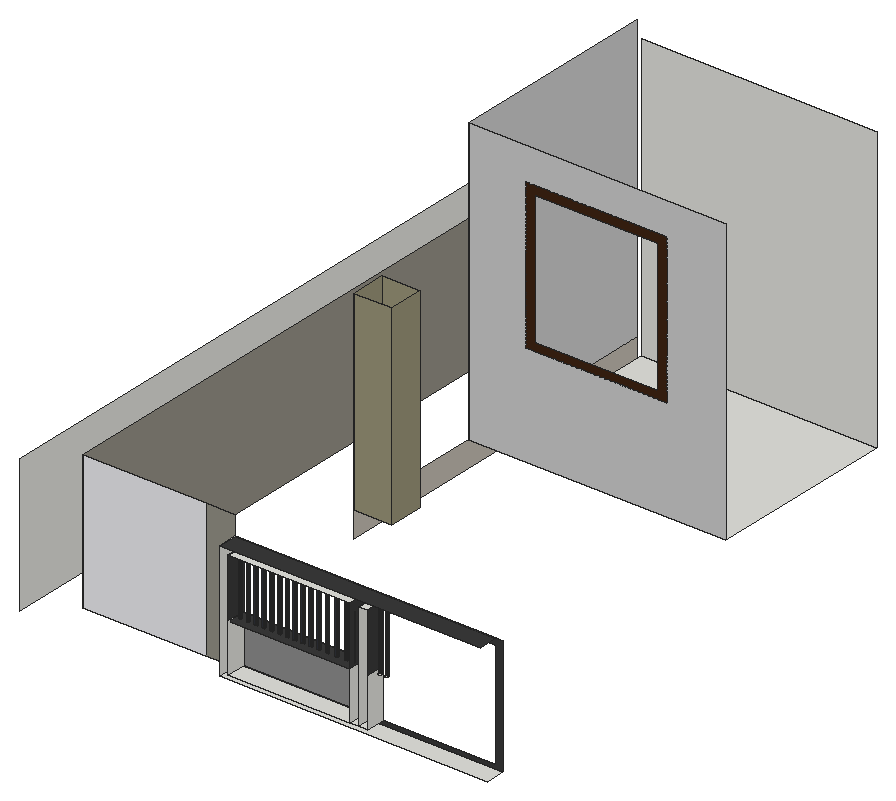
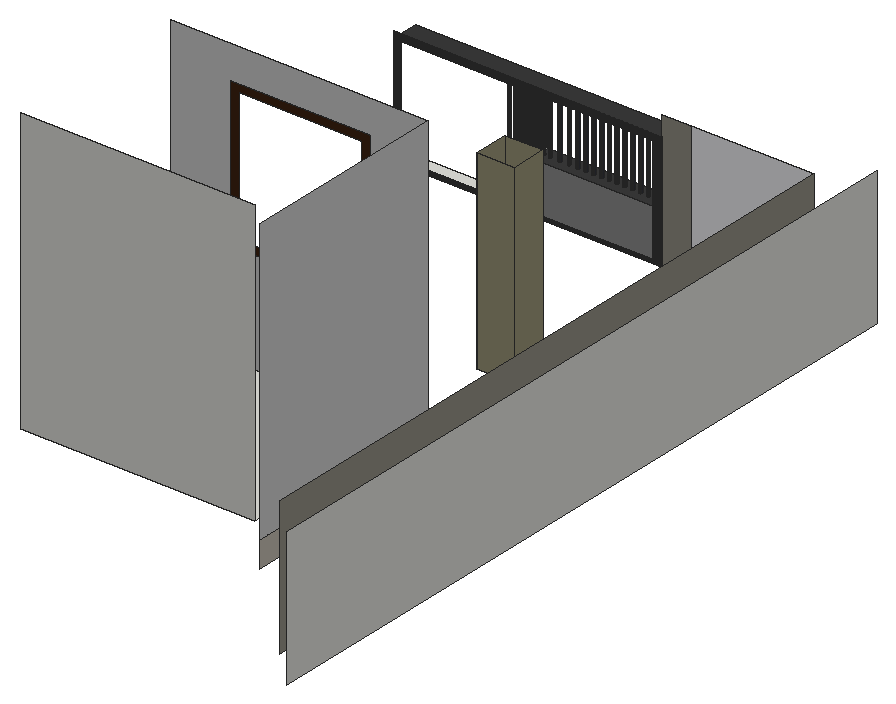
# SketchUp Ruby script. Lengths in inches.
U = 1.inch
M = Sketchup.active_model
def pt(a) = Geom::Point3d.new(a.map { |v| v * U })
def face(e, loops, mat)
  f = e.add_face(loops[0].map { |a| pt(a) })
  loops[1..].each { |l| e.add_face(l.map { |a| pt(a) }).erase! }
  f.material = f.back_material = mat if mat
  f
end
# faces: each face lists its corners as indices into pts; further lists are holes
def faces(e, pts, list, mat = nil) = list.each { |f| face(e, (f[0].is_a?(Array) ? f : [f]).map { |l| l.map { |i| pts[i] } }, mat) }
# xy, xz, yz: faces in a plane at the given z, y or x. An outline is a flat list of corners, or four numbers for a rectangle; further outlines are holes
def ring(l) = l.size == 4 ? [[l[0], l[1]], [l[2], l[1]], [l[2], l[3]], [l[0], l[3]]] : l.each_slice(2).to_a
def flat(e, list, mat, &to3) = list.each { |f| face(e, (f[0].is_a?(Array) ? f : [f]).map { |l| ring(l).map { |u, v| to3.(u, v) } }, mat) }
def xy(e, z, list, mat = nil) = flat(e, list, mat) { |x, y| [x, y, z] }
def xz(e, y, list, mat = nil) = flat(e, list, mat) { |x, z| [x, y, z] }
def yz(e, x, list, mat = nil) = flat(e, list, mat) { |y, z| [x, y, z] }
def lines(e, pts, list) = list.each { |a, b| e.add_line(pt(pts[a]), pt(pts[b])) }
# prism: a flat outline (further loops are holes) pulled along v
def prism(e, loops, v, mat = nil)
  f = face(e, loops, mat); d = Geom::Vector3d.new(v.map { |x| x * U })
  f.pushpull(f.normal.samedirection?(d) ? d.length : -d.length)
end
def box(e, o, s, mat = nil) = prism(e, [[o, [o[0] + s[0], o[1], o[2]], [o[0] + s[0], o[1] + s[1], o[2]], [o[0], o[1] + s[1], o[2]]]], [0, 0, s[2]], mat)
def at(x, y, z, deg = 0) = Geom::Transformation.translation(pt([x, y, z])) * Geom::Transformation.rotation(ORIGIN, Z_AXIS, deg.degrees)
def axes(o, x, y, z) = Geom::Transformation.new([*x, 0, *y, 0, *z, 0, *pt(o).to_a, 1])
def part(name) = M.definitions.add(name)
# library, detail: a bought-in or finely detailed component or shape, given as its bounding box
def library(name, o, s) = part(name).tap { |d| box(d.entities, o, s) }
def detail(e, o, s) = box(e.add_group.entities, o, s)
def put(e, d, t, mat = nil) = e.add_instance(d, t).tap { |i| i.material = mat if mat }
def group(e, t, mat = nil) = e.add_group.tap { |g| g.transformation = t; g.material = mat if mat }.entities
root = M.entities
M.materials.add("[Blinds Vertical Pattern]1").color = [239, 239, 242]
M.materials.add("[Cladding Siding White]").color = [207, 207, 207]
M.materials.add("[Color M04]").color = [142, 142, 142]
M.materials.add("[Color M07]").color = [58, 58, 58]
M.materials.add("[Field Rectangle Tile]").color = [196, 189, 179]
M.materials.add("[Formica Graystone]").color = [149, 146, 135]
M.materials.add("[Formica Laminate Dark]").color = [50, 53, 60]
M.materials.add("[Stone Coursed Rough]").color = [155, 150, 122]
M.materials.add("[Wood Veneer 01]").color = [63, 37, 19]
xy(root,0,[[79.1,102.91,192.64,111]])
xy(root,1.75,[[82.65,102.91,134.27,111],[134.27,102.91,138.0625,111],[138.0625,102.91,141.86,111]])
xy(root,10.875,[[55.77,203.17,71.76,217.98],[64.9,263.99,164.37,343.79]])
xy(root,22.1875,[[132.58,106,132.4,106.02,132.24,106.09,132.1,106.2,131.99,106.34,131.92,106.51,131.9,106.6875,131.92,106.87,131.99,107.03,132.1,107.17,132.24,107.28,132.4,107.35,132.58,107.375,132.76,107.35,132.93,107.28,133.07,107.17,133.18,107.03,133.25,106.87,133.27,106.6875,133.25,106.51,133.18,106.34,133.07,106.2,132.93,106.09,132.76,106.02],[144.08,106,143.9,106.02,143.74,106.09,143.6,106.2,143.49,106.34,143.42,106.51,143.4,106.6875,143.42,106.87,143.49,107.03,143.6,107.17,143.74,107.28,143.9,107.35,144.08,107.375,144.26,107.35,144.43,107.28,144.57,107.17,144.68,107.03,144.75,106.87,144.77,106.6875,144.75,106.51,144.68,106.34,144.57,106.2,144.43,106.09,144.26,106.02],[146.96,106,146.78,106.02,146.61,106.09,146.47,106.2,146.36,106.34,146.29,106.51,146.27,106.6875,146.29,106.87,146.36,107.03,146.47,107.17,146.61,107.28,146.78,107.35,146.96,107.375,147.14,107.35,147.3,107.28,147.44,107.17,147.55,107.03,147.62,106.87,147.65,106.6875,147.62,106.51,147.55,106.34,147.44,106.2,147.3,106.09,147.14,106.02]])
xy(root,22.1875,[[[82.65,102.91,134.27,111],[88.02,106,87.84,106.02,87.68,106.09,87.53,106.2,87.42,106.34,87.36,106.51,87.33,106.6875,87.36,106.87,87.42,107.03,87.53,107.17,87.68,107.28,87.84,107.35,88.02,107.375,88.2,107.35,88.36,107.28,88.51,107.17,88.62,107.03,88.68,106.87,88.71,106.6875,88.68,106.51,88.62,106.34,88.51,106.2,88.36,106.09,88.2,106.02],[91.33,106,91.15,106.02,90.99,106.09,90.85,106.2,90.74,106.34,90.67,106.51,90.65,106.6875,90.67,106.87,90.74,107.03,90.85,107.17,90.99,107.28,91.15,107.35,91.33,107.375,91.51,107.35,91.68,107.28,91.82,107.17,91.93,107.03,92,106.87,92.02,106.6875,92,106.51,91.93,106.34,91.82,106.2,91.68,106.09,91.51,106.02],[94.65,106,94.47,106.02,94.3,106.09,94.16,106.2,94.05,106.34,93.98,106.51,93.96,106.6875,93.98,106.87,94.05,107.03,94.16,107.17,94.3,107.28,94.47,107.35,94.65,107.375,94.82,107.35,94.99,107.28,95.13,107.17,95.24,107.03,95.31,106.87,95.33,106.6875,95.31,106.51,95.24,106.34,95.13,106.2,94.99,106.09,94.82,106.02],[97.96,106,97.78,106.02,97.61,106.09,97.47,106.2,97.36,106.34,97.29,106.51,97.27,106.6875,97.29,106.87,97.36,107.03,97.47,107.17,97.61,107.28,97.78,107.35,97.96,107.375,98.14,107.35,98.3,107.28,98.44,107.17,98.55,107.03,98.62,106.87,98.65,106.6875,98.62,106.51,98.55,106.34,98.44,106.2,98.3,106.09,98.14,106.02],[101.27,106,101.09,106.02,100.93,106.09,100.78,106.2,100.67,106.34,100.61,106.51,100.58,106.6875,100.61,106.87,100.67,107.03,100.78,107.17,100.93,107.28,101.09,107.35,101.27,107.375,101.45,107.35,101.61,107.28,101.76,107.17,101.87,107.03,101.93,106.87,101.96,106.6875,101.93,106.51,101.87,106.34,101.76,106.2,101.61,106.09,101.45,106.02],[104.58,106,104.4,106.02,104.24,106.09,104.1,106.2,103.99,106.34,103.92,106.51,103.9,106.6875,103.92,106.87,103.99,107.03,104.1,107.17,104.24,107.28,104.4,107.35,104.58,107.375,104.76,107.35,104.93,107.28,105.07,107.17,105.18,107.03,105.25,106.87,105.27,106.6875,105.25,106.51,105.18,106.34,105.07,106.2,104.93,106.09,104.76,106.02],[107.9,106,107.72,106.02,107.55,106.09,107.41,106.2,107.3,106.34,107.23,106.51,107.21,106.6875,107.23,106.87,107.3,107.03,107.41,107.17,107.55,107.28,107.72,107.35,107.9,107.375,108.07,107.35,108.24,107.28,108.38,107.17,108.49,107.03,108.56,106.87,108.58,106.6875,108.56,106.51,108.49,106.34,108.38,106.2,108.24,106.09,108.07,106.02],[111.21,106,111.03,106.02,110.86,106.09,110.72,106.2,110.61,106.34,110.54,106.51,110.52,106.6875,110.54,106.87,110.61,107.03,110.72,107.17,110.86,107.28,111.03,107.35,111.21,107.375,111.39,107.35,111.55,107.28,111.69,107.17,111.8,107.03,111.87,106.87,111.9,106.6875,111.87,106.51,111.8,106.34,111.69,106.2,111.55,106.09,111.39,106.02],[114.52,106,114.34,106.02,114.18,106.09,114.03,106.2,113.92,106.34,113.86,106.51,113.83,106.6875,113.86,106.87,113.92,107.03,114.03,107.17,114.18,107.28,114.34,107.35,114.52,107.375,114.7,107.35,114.86,107.28,115.01,107.17,115.12,107.03,115.18,106.87,115.21,106.6875,115.18,106.51,115.12,106.34,115.01,106.2,114.86,106.09,114.7,106.02],[132.58,106,132.4,106.02,132.24,106.09,132.1,106.2,131.99,106.34,131.92,106.51,131.9,106.6875,131.92,106.87,131.99,107.03,132.1,107.17,132.24,107.28,132.4,107.35,132.58,107.375,132.76,107.35,132.93,107.28,133.07,107.17,133.18,107.03,133.25,106.87,133.27,106.6875,133.25,106.51,133.18,106.34,133.07,106.2,132.93,106.09,132.76,106.02],[117.96,106,117.78,106.02,117.61,106.09,117.47,106.2,117.36,106.34,117.29,106.51,117.27,106.6875,117.29,106.87,117.36,107.03,117.47,107.17,117.61,107.28,117.78,107.35,117.96,107.375,118.14,107.35,118.3,107.28,118.44,107.17,118.55,107.03,118.62,106.87,118.65,106.6875,118.62,106.51,118.55,106.34,118.44,106.2,118.3,106.09,118.14,106.02],[129.58,106,129.4,106.02,129.24,106.09,129.1,106.2,128.99,106.34,128.92,106.51,128.9,106.6875,128.92,106.87,128.99,107.03,129.1,107.17,129.24,107.28,129.4,107.35,129.58,107.375,129.76,107.35,129.93,107.28,130.07,107.17,130.18,107.03,130.25,106.87,130.27,106.6875,130.25,106.51,130.18,106.34,130.07,106.2,129.93,106.09,129.76,106.02],[121.58,106,121.4,106.02,121.24,106.09,121.1,106.2,120.99,106.34,120.92,106.51,120.9,106.6875,120.92,106.87,120.99,107.03,121.1,107.17,121.24,107.28,121.4,107.35,121.58,107.375,121.76,107.35,121.93,107.28,122.07,107.17,122.18,107.03,122.25,106.87,122.27,106.6875,122.25,106.51,122.18,106.34,122.07,106.2,121.93,106.09,121.76,106.02],[125.52,106,125.34,106.02,125.18,106.09,125.03,106.2,124.92,106.34,124.86,106.51,124.83,106.6875,124.86,106.87,124.92,107.03,125.03,107.17,125.18,107.28,125.34,107.35,125.52,107.375,125.7,107.35,125.86,107.28,126.01,107.17,126.12,107.03,126.18,106.87,126.21,106.6875,126.18,106.51,126.12,106.34,126.01,106.2,125.86,106.09,125.7,106.02],[84.71,106,84.53,106.02,84.36,106.09,84.22,106.2,84.11,106.34,84.04,106.51,84.02,106.6875,84.04,106.87,84.11,107.03,84.22,107.17,84.36,107.28,84.53,107.35,84.71,107.375,84.89,107.35,85.05,107.28,85.19,107.17,85.3,107.03,85.37,106.87,85.4,106.6875,85.37,106.51,85.3,106.34,85.19,106.2,85.05,106.09,84.89,106.02]]],"[Color M07]")
xy(root,47.21,[[[82.65,102.91,134.27,111],[84.71,106,84.89,106.02,85.05,106.09,85.19,106.2,85.3,106.34,85.37,106.51,85.4,106.6875,85.37,106.87,85.3,107.03,85.19,107.17,85.05,107.28,84.89,107.35,84.71,107.375,84.53,107.35,84.36,107.28,84.22,107.17,84.11,107.03,84.04,106.87,84.02,106.6875,84.04,106.51,84.11,106.34,84.22,106.2,84.36,106.09,84.53,106.02],[88.02,106,88.2,106.02,88.36,106.09,88.51,106.2,88.62,106.34,88.68,106.51,88.71,106.6875,88.68,106.87,88.62,107.03,88.51,107.17,88.36,107.28,88.2,107.35,88.02,107.375,87.84,107.35,87.68,107.28,87.53,107.17,87.42,107.03,87.36,106.87,87.33,106.6875,87.36,106.51,87.42,106.34,87.53,106.2,87.68,106.09,87.84,106.02],[91.33,106,91.51,106.02,91.68,106.09,91.82,106.2,91.93,106.34,92,106.51,92.02,106.6875,92,106.87,91.93,107.03,91.82,107.17,91.68,107.28,91.51,107.35,91.33,107.375,91.15,107.35,90.99,107.28,90.85,107.17,90.74,107.03,90.67,106.87,90.65,106.6875,90.67,106.51,90.74,106.34,90.85,106.2,90.99,106.09,91.15,106.02],[94.65,106,94.82,106.02,94.99,106.09,95.13,106.2,95.24,106.34,95.31,106.51,95.33,106.6875,95.31,106.87,95.24,107.03,95.13,107.17,94.99,107.28,94.82,107.35,94.65,107.375,94.47,107.35,94.3,107.28,94.16,107.17,94.05,107.03,93.98,106.87,93.96,106.6875,93.98,106.51,94.05,106.34,94.16,106.2,94.3,106.09,94.47,106.02],[97.96,106,98.14,106.02,98.3,106.09,98.44,106.2,98.55,106.34,98.62,106.51,98.65,106.6875,98.62,106.87,98.55,107.03,98.44,107.17,98.3,107.28,98.14,107.35,97.96,107.375,97.78,107.35,97.61,107.28,97.47,107.17,97.36,107.03,97.29,106.87,97.27,106.6875,97.29,106.51,97.36,106.34,97.47,106.2,97.61,106.09,97.78,106.02],[101.27,106,101.45,106.02,101.61,106.09,101.76,106.2,101.87,106.34,101.93,106.51,101.96,106.6875,101.93,106.87,101.87,107.03,101.76,107.17,101.61,107.28,101.45,107.35,101.27,107.375,101.09,107.35,100.93,107.28,100.78,107.17,100.67,107.03,100.61,106.87,100.58,106.6875,100.61,106.51,100.67,106.34,100.78,106.2,100.93,106.09,101.09,106.02],[104.58,106,104.76,106.02,104.93,106.09,105.07,106.2,105.18,106.34,105.25,106.51,105.27,106.6875,105.25,106.87,105.18,107.03,105.07,107.17,104.93,107.28,104.76,107.35,104.58,107.375,104.4,107.35,104.24,107.28,104.1,107.17,103.99,107.03,103.92,106.87,103.9,106.6875,103.92,106.51,103.99,106.34,104.1,106.2,104.24,106.09,104.4,106.02],[107.9,106,108.07,106.02,108.24,106.09,108.38,106.2,108.49,106.34,108.56,106.51,108.58,106.6875,108.56,106.87,108.49,107.03,108.38,107.17,108.24,107.28,108.07,107.35,107.9,107.375,107.72,107.35,107.55,107.28,107.41,107.17,107.3,107.03,107.23,106.87,107.21,106.6875,107.23,106.51,107.3,106.34,107.41,106.2,107.55,106.09,107.72,106.02],[111.21,106,111.39,106.02,111.55,106.09,111.69,106.2,111.8,106.34,111.87,106.51,111.9,106.6875,111.87,106.87,111.8,107.03,111.69,107.17,111.55,107.28,111.39,107.35,111.21,107.375,111.03,107.35,110.86,107.28,110.72,107.17,110.61,107.03,110.54,106.87,110.52,106.6875,110.54,106.51,110.61,106.34,110.72,106.2,110.86,106.09,111.03,106.02],[114.52,106,114.7,106.02,114.86,106.09,115.01,106.2,115.12,106.34,115.18,106.51,115.21,106.6875,115.18,106.87,115.12,107.03,115.01,107.17,114.86,107.28,114.7,107.35,114.52,107.375,114.34,107.35,114.18,107.28,114.03,107.17,113.92,107.03,113.86,106.87,113.83,106.6875,113.86,106.51,113.92,106.34,114.03,106.2,114.18,106.09,114.34,106.02],[117.96,106,118.14,106.02,118.3,106.09,118.44,106.2,118.55,106.34,118.62,106.51,118.65,106.6875,118.62,106.87,118.55,107.03,118.44,107.17,118.3,107.28,118.14,107.35,117.96,107.375,117.78,107.35,117.61,107.28,117.47,107.17,117.36,107.03,117.29,106.87,117.27,106.6875,117.29,106.51,117.36,106.34,117.47,106.2,117.61,106.09,117.78,106.02],[121.58,106,121.76,106.02,121.93,106.09,122.07,106.2,122.18,106.34,122.25,106.51,122.27,106.6875,122.25,106.87,122.18,107.03,122.07,107.17,121.93,107.28,121.76,107.35,121.58,107.375,121.4,107.35,121.24,107.28,121.1,107.17,120.99,107.03,120.92,106.87,120.9,106.6875,120.92,106.51,120.99,106.34,121.1,106.2,121.24,106.09,121.4,106.02],[125.52,106,125.7,106.02,125.86,106.09,126.01,106.2,126.12,106.34,126.18,106.51,126.21,106.6875,126.18,106.87,126.12,107.03,126.01,107.17,125.86,107.28,125.7,107.35,125.52,107.375,125.34,107.35,125.18,107.28,125.03,107.17,124.92,107.03,124.86,106.87,124.83,106.6875,124.86,106.51,124.92,106.34,125.03,106.2,125.18,106.09,125.34,106.02],[129.58,106,129.76,106.02,129.93,106.09,130.07,106.2,130.18,106.34,130.25,106.51,130.27,106.6875,130.25,106.87,130.18,107.03,130.07,107.17,129.93,107.28,129.76,107.35,129.58,107.375,129.4,107.35,129.24,107.28,129.1,107.17,128.99,107.03,128.92,106.87,128.9,106.6875,128.92,106.51,128.99,106.34,129.1,106.2,129.24,106.09,129.4,106.02],[132.58,106,132.76,106.02,132.93,106.09,133.07,106.2,133.18,106.34,133.25,106.51,133.27,106.6875,133.25,106.87,133.18,107.03,133.07,107.17,132.93,107.28,132.76,107.35,132.58,107.375,132.4,107.35,132.24,107.28,132.1,107.17,131.99,107.03,131.92,106.87,131.9,106.6875,131.92,106.51,131.99,106.34,132.1,106.2,132.24,106.09,132.4,106.02]],[138.0625,102.91,141.86,111]])
xy(root,49.625,[[79.1,102.91,189.5,111]],"[Color M07]")
xz(root,111,[[14.76,0,66.82,57.8125]],"[Blinds Vertical Pattern]1")
xz(root,111,[[82.65,1.75,134.27,22.1875]],"[Color M04]")
xz(root,111,[[[79.1,0,192.64,49.625],[82.65,1.75,189.5,47.21]],[134.27,1.75,138.0625,47.21],[138.0625,1.75,141.86,47.21]],"[Color M07]")
xz(root,111,[[66.82,0,79.1,57.8125]],"[Formica Graystone]")
xz(root,203.17,[[55.77,10.875,71.76,93.02]],"[Stone Coursed Rough]")
xz(root,217.98,[[55.77,10.875,71.76,93.02]],"[Stone Coursed Rough]")
xz(root,263.99,[[[55.77,10.875,164.37,130.875],[80,53.99,139.3125,117.05]]],"[Cladding Siding White]")
xz(root,263.99,[[[80,53.99,139.3125,117.05],[83.47,57.46,135.84,113.58]]],"[Wood Veneer 01]")
xz(root,343.79,[[64.9,10.875,164.37,130.875]])
yz(root,0,[[96.24,0,408.18,57.8125]])
yz(root,14.76,[[111,0,393.42,57.8125]],"[Formica Graystone]")
yz(root,55.77,[[263.99,10.875,352.92,130.875]],"[Cladding Siding White]")
yz(root,55.77,[[203.17,0,352.92,10.875]],"[Field Rectangle Tile]")
yz(root,55.77,[[203.17,10.875,217.98,93.02]],"[Stone Coursed Rough]")
yz(root,71.76,[[203.17,10.875,217.98,93.02]],"[Stone Coursed Rough]")
yz(root,79.1,[[102.91,0,111,49.625]])
yz(root,82.65,[[102.91,1.75,111,22.1875]])
yz(root,82.65,[[102.91,22.1875,111,47.21]],"[Color M07]")
yz(root,134.27,[[102.91,1.75,111,22.1875]])
yz(root,134.27,[[102.91,22.1875,111,47.21]],"[Color M07]")
yz(root,138.0625,[[102.91,1.75,111,47.21]])
yz(root,141.86,[[102.91,1.75,111,22.1875]])
yz(root,141.86,[[102.91,22.1875,111,47.21]],"[Color M07]")
p = [[84.04,106.87,22.1875],[84.02,106.6875,22.1875],[84.02,106.6875,47.21],[84.04,106.87,47.21],[85.4,106.6875,22.1875],[85.37,106.87,22.1875],
  [85.37,106.87,47.21],[85.4,106.6875,47.21],[87.36,106.87,22.1875],[87.33,106.6875,22.1875],[87.33,106.6875,47.21],[87.36,106.87,47.21],
  [88.71,106.6875,22.1875],[88.68,106.87,22.1875],[88.68,106.87,47.21],[88.71,106.6875,47.21],[90.67,106.87,22.1875],[90.65,106.6875,22.1875],
  [90.65,106.6875,47.21],[90.67,106.87,47.21],[92.02,106.6875,22.1875],[92,106.87,22.1875],[92,106.87,47.21],[92.02,106.6875,47.21],
  [93.98,106.87,22.1875],[93.96,106.6875,22.1875],[93.96,106.6875,47.21],[93.98,106.87,47.21],[95.33,106.6875,22.1875],[95.31,106.87,22.1875],
  [95.31,106.87,47.21],[95.33,106.6875,47.21],[97.29,106.87,22.1875],[97.27,106.6875,22.1875],[97.27,106.6875,47.21],[97.29,106.87,47.21],
  [98.65,106.6875,22.1875],[98.62,106.87,22.1875],[98.62,106.87,47.21],[98.65,106.6875,47.21],[100.61,106.87,22.1875],[100.58,106.6875,22.1875],
  [100.58,106.6875,47.21],[100.61,106.87,47.21],[101.96,106.6875,22.1875],[101.93,106.87,22.1875],[101.93,106.87,47.21],[101.96,106.6875,47.21],
  [103.92,106.87,22.1875],[103.9,106.6875,22.1875],[103.9,106.6875,47.21],[103.92,106.87,47.21],[105.27,106.6875,22.1875],[105.25,106.87,22.1875],
  [105.25,106.87,47.21],[105.27,106.6875,47.21],[107.23,106.87,22.1875],[107.21,106.6875,22.1875],[107.21,106.6875,47.21],[107.23,106.87,47.21],
  [108.58,106.6875,22.1875],[108.56,106.87,22.1875],[108.56,106.87,47.21],[108.58,106.6875,47.21],[110.54,106.87,22.1875],[110.52,106.6875,22.1875],
  [110.52,106.6875,47.21],[110.54,106.87,47.21],[111.9,106.6875,22.1875],[111.87,106.87,22.1875],[111.87,106.87,47.21],[111.9,106.6875,47.21],
  [113.86,106.87,22.1875],[113.83,106.6875,22.1875],[113.83,106.6875,47.21],[113.86,106.87,47.21],[115.21,106.6875,22.1875],[115.18,106.87,22.1875],
  [115.18,106.87,47.21],[115.21,106.6875,47.21],[117.29,106.87,22.1875],[117.27,106.6875,22.1875],[117.27,106.6875,47.21],[117.29,106.87,47.21],
  [118.65,106.6875,22.1875],[118.62,106.87,22.1875],[118.62,106.87,47.21],[118.65,106.6875,47.21],[120.92,106.87,22.1875],[120.9,106.6875,22.1875],
  [120.9,106.6875,47.21],[120.92,106.87,47.21],[122.27,106.6875,22.1875],[122.25,106.87,22.1875],[122.25,106.87,47.21],[122.27,106.6875,47.21],
  [124.86,106.87,22.1875],[124.83,106.6875,22.1875],[124.83,106.6875,47.21],[124.86,106.87,47.21],[126.21,106.6875,22.1875],[126.18,106.87,22.1875],
  [126.18,106.87,47.21],[126.21,106.6875,47.21],[128.92,106.87,22.1875],[128.9,106.6875,22.1875],[128.9,106.6875,47.21],[128.92,106.87,47.21],
  [130.27,106.6875,22.1875],[130.25,106.87,22.1875],[130.25,106.87,47.21],[130.27,106.6875,47.21],[131.92,106.87,22.1875],[131.9,106.6875,22.1875],
  [131.9,106.6875,47.21],[131.92,106.87,47.21],[133.27,106.6875,22.1875],[133.25,106.87,22.1875],[133.25,106.87,47.21],[133.27,106.6875,47.21],
  [143.42,106.87,22.1875],[143.4,106.6875,22.1875],[143.4,106.6875,47.21],[143.42,106.87,47.21],[144.77,106.6875,22.1875],[144.75,106.87,22.1875],
  [144.75,106.87,47.21],[144.77,106.6875,47.21],[146.29,106.87,22.1875],[146.27,106.6875,22.1875],[146.27,106.6875,47.21],[146.29,106.87,47.21],
  [84.11,107.03,22.1875],[84.11,107.03,47.21],[85.3,107.03,22.1875],[85.3,107.03,47.21],[87.42,107.03,22.1875],[87.42,107.03,47.21],
  [88.62,107.03,22.1875],[88.62,107.03,47.21],[90.74,107.03,22.1875],[90.74,107.03,47.21],[91.93,107.03,22.1875],[91.93,107.03,47.21],
  [94.05,107.03,22.1875],[94.05,107.03,47.21],[95.24,107.03,22.1875],[95.24,107.03,47.21],[97.36,107.03,22.1875],[97.36,107.03,47.21],
  [98.55,107.03,22.1875],[98.55,107.03,47.21],[100.67,107.03,22.1875],[100.67,107.03,47.21],[101.87,107.03,22.1875],[101.87,107.03,47.21],
  [103.99,107.03,22.1875],[103.99,107.03,47.21],[105.18,107.03,22.1875],[105.18,107.03,47.21],[107.3,107.03,22.1875],[107.3,107.03,47.21],
  [108.49,107.03,22.1875],[108.49,107.03,47.21],[110.61,107.03,22.1875],[110.61,107.03,47.21],[111.8,107.03,22.1875],[111.8,107.03,47.21],
  [113.92,107.03,22.1875],[113.92,107.03,47.21],[115.12,107.03,22.1875],[115.12,107.03,47.21],[117.36,107.03,22.1875],[117.36,107.03,47.21],
  [118.55,107.03,22.1875],[118.55,107.03,47.21],[120.99,107.03,22.1875],[120.99,107.03,47.21],[122.18,107.03,22.1875],[122.18,107.03,47.21],
  [124.92,107.03,22.1875],[124.92,107.03,47.21],[126.12,107.03,22.1875],[126.12,107.03,47.21],[128.99,107.03,22.1875],[128.99,107.03,47.21],
  [130.18,107.03,22.1875],[130.18,107.03,47.21],[131.99,107.03,22.1875],[131.99,107.03,47.21],[133.18,107.03,22.1875],[133.18,107.03,47.21],
  [143.49,107.03,22.1875],[143.49,107.03,47.21],[144.68,107.03,22.1875],[144.68,107.03,47.21],[146.36,107.03,22.1875],[146.36,107.03,47.21],
  [84.22,107.17,22.1875],[84.22,107.17,47.21],[85.19,107.17,22.1875],[85.19,107.17,47.21],[87.53,107.17,22.1875],[87.53,107.17,47.21],
  [88.51,107.17,22.1875],[88.51,107.17,47.21],[90.85,107.17,22.1875],[90.85,107.17,47.21],[91.82,107.17,22.1875],[91.82,107.17,47.21],
  [94.16,107.17,22.1875],[94.16,107.17,47.21],[95.13,107.17,22.1875],[95.13,107.17,47.21],[97.47,107.17,22.1875],[97.47,107.17,47.21],
  [98.44,107.17,22.1875],[98.44,107.17,47.21],[100.78,107.17,22.1875],[100.78,107.17,47.21],[101.76,107.17,22.1875],[101.76,107.17,47.21],
  [104.1,107.17,22.1875],[104.1,107.17,47.21],[105.07,107.17,22.1875],[105.07,107.17,47.21],[107.41,107.17,22.1875],[107.41,107.17,47.21],
  [108.38,107.17,22.1875],[108.38,107.17,47.21],[110.72,107.17,22.1875],[110.72,107.17,47.21],[111.69,107.17,22.1875],[111.69,107.17,47.21],
  [114.03,107.17,22.1875],[114.03,107.17,47.21],[115.01,107.17,22.1875],[115.01,107.17,47.21],[117.47,107.17,22.1875],[117.47,107.17,47.21],
  [118.44,107.17,22.1875],[118.44,107.17,47.21],[121.1,107.17,22.1875],[121.1,107.17,47.21],[122.07,107.17,22.1875],[122.07,107.17,47.21],
  [125.03,107.17,22.1875],[125.03,107.17,47.21],[126.01,107.17,22.1875],[126.01,107.17,47.21],[129.1,107.17,22.1875],[129.1,107.17,47.21],
  [130.07,107.17,22.1875],[130.07,107.17,47.21],[132.1,107.17,22.1875],[132.1,107.17,47.21],[133.07,107.17,22.1875],[133.07,107.17,47.21],
  [143.6,107.17,22.1875],[143.6,107.17,47.21],[144.57,107.17,22.1875],[144.57,107.17,47.21],[146.47,107.17,22.1875],[146.47,107.17,47.21],
  [84.36,107.28,22.1875],[84.36,107.28,47.21],[85.05,107.28,22.1875],[85.05,107.28,47.21],[87.68,107.28,22.1875],[87.68,107.28,47.21],
  [88.36,107.28,22.1875],[88.36,107.28,47.21],[90.99,107.28,22.1875],[90.99,107.28,47.21],[91.68,107.28,22.1875],[91.68,107.28,47.21],
  [94.3,107.28,22.1875],[94.3,107.28,47.21],[94.99,107.28,22.1875],[94.99,107.28,47.21],[97.61,107.28,22.1875],[97.61,107.28,47.21],
  [98.3,107.28,22.1875],[98.3,107.28,47.21],[100.93,107.28,22.1875],[100.93,107.28,47.21],[101.61,107.28,22.1875],[101.61,107.28,47.21],
  [104.24,107.28,22.1875],[104.24,107.28,47.21],[104.93,107.28,22.1875],[104.93,107.28,47.21],[107.55,107.28,22.1875],[107.55,107.28,47.21],
  [108.24,107.28,22.1875],[108.24,107.28,47.21],[110.86,107.28,22.1875],[110.86,107.28,47.21],[111.55,107.28,22.1875],[111.55,107.28,47.21],
  [114.18,107.28,22.1875],[114.18,107.28,47.21],[114.86,107.28,22.1875],[114.86,107.28,47.21],[117.61,107.28,22.1875],[117.61,107.28,47.21],
  [118.3,107.28,22.1875],[118.3,107.28,47.21],[121.24,107.28,22.1875],[121.24,107.28,47.21],[121.93,107.28,22.1875],[121.93,107.28,47.21],
  [125.18,107.28,22.1875],[125.18,107.28,47.21],[125.86,107.28,22.1875],[125.86,107.28,47.21],[129.24,107.28,22.1875],[129.24,107.28,47.21],
  [129.93,107.28,22.1875],[129.93,107.28,47.21],[132.24,107.28,22.1875],[132.24,107.28,47.21],[132.93,107.28,22.1875],[132.93,107.28,47.21],
  [143.74,107.28,22.1875],[143.74,107.28,47.21],[144.43,107.28,22.1875],[144.43,107.28,47.21],[146.61,107.28,22.1875],[146.61,107.28,47.21],
  [84.53,107.35,22.1875],[84.53,107.35,47.21],[84.89,107.35,22.1875],[84.89,107.35,47.21],[87.84,107.35,22.1875],[87.84,107.35,47.21],
  [88.2,107.35,22.1875],[88.2,107.35,47.21],[91.15,107.35,22.1875],[91.15,107.35,47.21],[91.51,107.35,22.1875],[91.51,107.35,47.21],
  [94.47,107.35,22.1875],[94.47,107.35,47.21],[94.82,107.35,22.1875],[94.82,107.35,47.21],[97.78,107.35,22.1875],[97.78,107.35,47.21],
  [98.14,107.35,22.1875],[98.14,107.35,47.21],[101.09,107.35,22.1875],[101.09,107.35,47.21],[101.45,107.35,22.1875],[101.45,107.35,47.21],
  [104.4,107.35,22.1875],[104.4,107.35,47.21],[104.76,107.35,22.1875],[104.76,107.35,47.21],[107.72,107.35,22.1875],[107.72,107.35,47.21],
  [108.07,107.35,22.1875],[108.07,107.35,47.21],[111.03,107.35,22.1875],[111.03,107.35,47.21],[111.39,107.35,22.1875],[111.39,107.35,47.21],
  [114.34,107.35,22.1875],[114.34,107.35,47.21],[114.7,107.35,22.1875],[114.7,107.35,47.21],[117.78,107.35,22.1875],[117.78,107.35,47.21],
  [118.14,107.35,22.1875],[118.14,107.35,47.21],[121.4,107.35,22.1875],[121.4,107.35,47.21],[121.76,107.35,22.1875],[121.76,107.35,47.21],
  [125.34,107.35,22.1875],[125.34,107.35,47.21],[125.7,107.35,22.1875],[125.7,107.35,47.21],[129.4,107.35,22.1875],[129.4,107.35,47.21],
  [129.76,107.35,22.1875],[129.76,107.35,47.21],[132.4,107.35,22.1875],[132.4,107.35,47.21],[132.76,107.35,22.1875],[132.76,107.35,47.21],
  [143.9,107.35,22.1875],[143.9,107.35,47.21],[144.26,107.35,22.1875],[144.26,107.35,47.21],[146.78,107.35,22.1875],[146.78,107.35,47.21],
  [147.3,107.28,22.1875],[147.14,107.35,22.1875],[147.14,107.35,47.21],[147.3,107.28,47.21],[84.71,107.375,22.1875],[84.71,107.375,47.21],
  [88.02,107.375,22.1875],[88.02,107.375,47.21],[91.33,107.375,22.1875],[91.33,107.375,47.21],[94.65,107.375,22.1875],[94.65,107.375,47.21],
  [97.96,107.375,22.1875],[97.96,107.375,47.21],[101.27,107.375,22.1875],[101.27,107.375,47.21],[104.58,107.375,22.1875],[104.58,107.375,47.21],
  [107.9,107.375,22.1875],[107.9,107.375,47.21],[111.21,107.375,22.1875],[111.21,107.375,47.21],[114.52,107.375,22.1875],[114.52,107.375,47.21],
  [117.96,107.375,22.1875],[117.96,107.375,47.21],[121.58,107.375,22.1875],[121.58,107.375,47.21],[125.52,107.375,22.1875],[125.52,107.375,47.21],
  [129.58,107.375,22.1875],[129.58,107.375,47.21],[132.58,107.375,22.1875],[132.58,107.375,47.21],[144.08,107.375,22.1875],[144.08,107.375,47.21],
  [146.96,107.375,22.1875],[146.96,107.375,47.21]]
faces(root,p,[[0,1,2,3],[4,5,6,7],[8,9,10,11],[12,13,14,15],[16,17,18,19],[20,21,22,23],[24,25,26,27],[28,29,30,31],
  [32,33,34,35],[36,37,38,39],[40,41,42,43],[44,45,46,47],[48,49,50,51],[52,53,54,55],[56,57,58,59],[60,61,62,63],
  [64,65,66,67],[68,69,70,71],[72,73,74,75],[76,77,78,79],[80,81,82,83],[84,85,86,87],[88,89,90,91],[92,93,94,95],
  [96,97,98,99],[100,101,102,103],[104,105,106,107],[108,109,110,111],[112,113,114,115],[116,117,118,119],[120,121,122,123],[124,125,126,127],
  [128,129,130,131],[132,0,3,133],[5,134,135,6],[136,8,11,137],[13,138,139,14],[140,16,19,141],[21,142,143,22],[144,24,27,145],
  [29,146,147,30],[148,32,35,149],[37,150,151,38],[152,40,43,153],[45,154,155,46],[156,48,51,157],[53,158,159,54],[160,56,59,161],
  [61,162,163,62],[164,64,67,165],[69,166,167,70],[168,72,75,169],[77,170,171,78],[172,80,83,173],[85,174,175,86],[176,88,91,177],
  [93,178,179,94],[180,96,99,181],[101,182,183,102],[184,104,107,185],[109,186,187,110],[188,112,115,189],[117,190,191,118],[192,120,123,193],
  [125,194,195,126],[196,128,131,197],[198,132,133,199],[134,200,201,135],[202,136,137,203],[138,204,205,139],[206,140,141,207],[142,208,209,143],
  [210,144,145,211],[146,212,213,147],[214,148,149,215],[150,216,217,151],[218,152,153,219],[154,220,221,155],[222,156,157,223],[158,224,225,159],
  [226,160,161,227],[162,228,229,163],[230,164,165,231],[166,232,233,167],[234,168,169,235],[170,236,237,171],[238,172,173,239],[174,240,241,175],
  [242,176,177,243],[178,244,245,179],[246,180,181,247],[182,248,249,183],[250,184,185,251],[186,252,253,187],[254,188,189,255],[190,256,257,191],
  [258,192,193,259],[194,260,261,195],[262,196,197,263],[264,198,199,265],[200,266,267,201],[268,202,203,269],[204,270,271,205],[272,206,207,273],
  [208,274,275,209],[276,210,211,277],[212,278,279,213],[280,214,215,281],[216,282,283,217],[284,218,219,285],[220,286,287,221],[288,222,223,289],
  [224,290,291,225],[292,226,227,293],[228,294,295,229],[296,230,231,297],[232,298,299,233],[300,234,235,301],[236,302,303,237],[304,238,239,305],
  [240,306,307,241],[308,242,243,309],[244,310,311,245],[312,246,247,313],[248,314,315,249],[316,250,251,317],[252,318,319,253],[320,254,255,321],
  [256,322,323,257],[324,258,259,325],[260,326,327,261],[328,262,263,329],[330,264,265,331],[266,332,333,267],[334,268,269,335],[270,336,337,271],
  [338,272,273,339],[274,340,341,275],[342,276,277,343],[278,344,345,279],[346,280,281,347],[282,348,349,283],[350,284,285,351],[286,352,353,287],
  [354,288,289,355],[290,356,357,291],[358,292,293,359],[294,360,361,295],[362,296,297,363],[298,364,365,299],[366,300,301,367],[302,368,369,303],
  [370,304,305,371],[306,372,373,307],[374,308,309,375],[310,376,377,311],[378,312,313,379],[314,380,381,315],[382,316,317,383],[318,384,385,319],
  [386,320,321,387],[322,388,389,323],[390,324,325,391],[326,392,393,327],[394,328,329,395],[396,397,398,399],[400,330,331,401],[332,400,401,333],
  [402,334,335,403],[336,402,403,337],[404,338,339,405],[340,404,405,341],[406,342,343,407],[344,406,407,345],[408,346,347,409],[348,408,409,349],
  [410,350,351,411],[352,410,411,353],[412,354,355,413],[356,412,413,357],[414,358,359,415],[360,414,415,361],[416,362,363,417],[364,416,417,365],
  [418,366,367,419],[368,418,419,369],[420,370,371,421],[372,420,421,373],[422,374,375,423],[376,422,423,377],[424,378,379,425],[380,424,425,381],
  [426,382,383,427],[384,426,427,385],[428,386,387,429],[388,428,429,389],[430,390,391,431],[392,430,431,393],[432,394,395,433],[397,432,433,398]],"[Formica Laminate Dark]")
